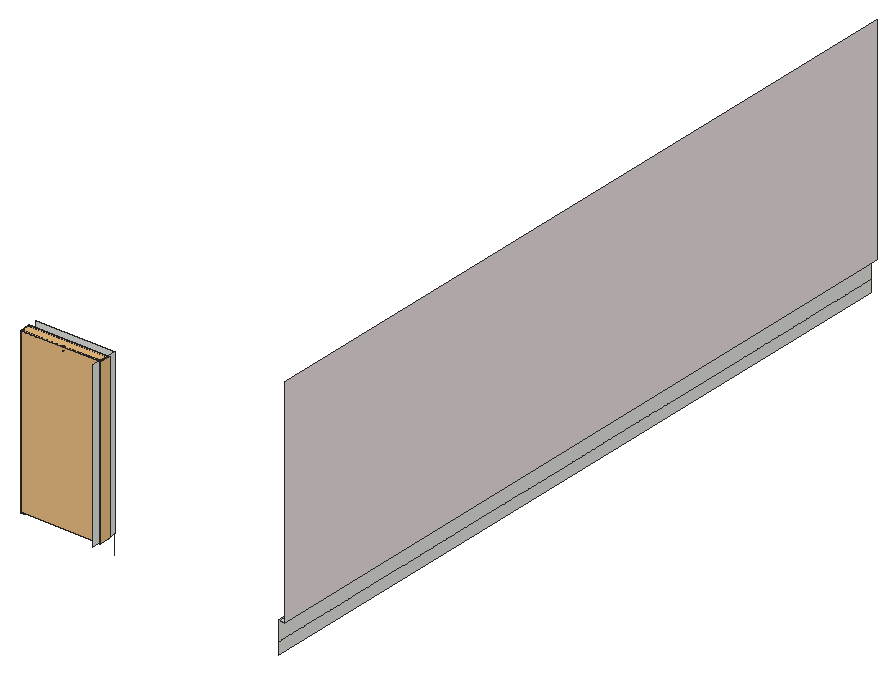
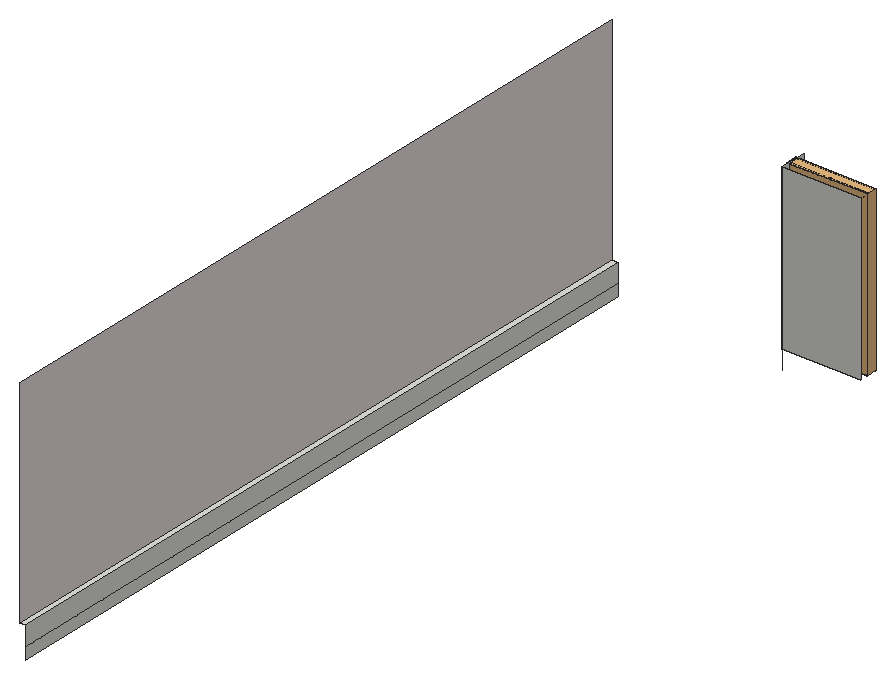
# SketchUp Ruby script. Lengths in inches.
U = 1.inch
M = Sketchup.active_model
def pt(a) = Geom::Point3d.new(a.map { |v| v * U })
def face(e, loops, mat)
  f = e.add_face(loops[0].map { |a| pt(a) })
  loops[1..].each { |l| e.add_face(l.map { |a| pt(a) }).erase! }
  f.material = f.back_material = mat if mat
  f
end
# faces: each face lists its corners as indices into pts; further lists are holes
def faces(e, pts, list, mat = nil) = list.each { |f| face(e, (f[0].is_a?(Array) ? f : [f]).map { |l| l.map { |i| pts[i] } }, mat) }
# xy, xz, yz: faces in a plane at the given z, y or x. An outline is a flat list of corners, or four numbers for a rectangle; further outlines are holes
def ring(l) = l.size == 4 ? [[l[0], l[1]], [l[2], l[1]], [l[2], l[3]], [l[0], l[3]]] : l.each_slice(2).to_a
def flat(e, list, mat, &to3) = list.each { |f| face(e, (f[0].is_a?(Array) ? f : [f]).map { |l| ring(l).map { |u, v| to3.(u, v) } }, mat) }
def xy(e, z, list, mat = nil) = flat(e, list, mat) { |x, y| [x, y, z] }
def xz(e, y, list, mat = nil) = flat(e, list, mat) { |x, z| [x, y, z] }
def yz(e, x, list, mat = nil) = flat(e, list, mat) { |y, z| [x, y, z] }
def lines(e, pts, list) = list.each { |a, b| e.add_line(pt(pts[a]), pt(pts[b])) }
# prism: a flat outline (further loops are holes) pulled along v
def prism(e, loops, v, mat = nil)
  f = face(e, loops, mat); d = Geom::Vector3d.new(v.map { |x| x * U })
  f.pushpull(f.normal.samedirection?(d) ? d.length : -d.length)
end
def box(e, o, s, mat = nil) = prism(e, [[o, [o[0] + s[0], o[1], o[2]], [o[0] + s[0], o[1] + s[1], o[2]], [o[0], o[1] + s[1], o[2]]]], [0, 0, s[2]], mat)
def at(x, y, z, deg = 0) = Geom::Transformation.translation(pt([x, y, z])) * Geom::Transformation.rotation(ORIGIN, Z_AXIS, deg.degrees)
def axes(o, x, y, z) = Geom::Transformation.new([*x, 0, *y, 0, *z, 0, *pt(o).to_a, 1])
def part(name) = M.definitions.add(name)
# library, detail: a bought-in or finely detailed component or shape, given as its bounding box
def library(name, o, s) = part(name).tap { |d| box(d.entities, o, s) }
def detail(e, o, s) = box(e.add_group.entities, o, s)
def put(e, d, t, mat = nil) = e.add_instance(d, t).tap { |i| i.material = mat if mat }
def group(e, t, mat = nil) = e.add_group.tap { |g| g.transformation = t; g.material = mat if mat }.entities
root = M.entities
M.materials.add("Generic\#9").color = [233, 223, 223]
M.materials.add("Material \#0").color = [86, 53, 35]
M.materials.add("Material \#1").color = [140, 140, 140]
c1 = part("3DGeom~19_Defintion")
xy(c1.entities,0,[[-6.28,-215.79,-994.45,-208.55,-13.52,-208.55],[-994.45,-215.79,-994.45,-208.55,-6.28,-215.79],[-6.28,-215.79,-13.52,-208.55,-13.52,0],[-6.28,-215.79,-13.52,0,-6.28,0],[-13.52,0,-13.52,208.55,-6.28,215.79],
  [-13.52,0,-6.28,215.79,-6.28,0],[-994.45,208.55,-6.28,215.79,-13.52,208.55],[-994.45,208.55,-994.45,215.79,-6.28,215.79]],"Material \#0")
p = [[-13.52,-208.55,0],[-994.45,-208.55,0],[-994.45,-207.81,0.07],[-14.25,-207.81,0.07],[-13.52,-208.55,0],[-14.25,-207.81,0.07],
  [-14.25,0,0.07],[-13.52,0,0],[-13.52,208.55,0],[-14.25,207.81,0.07],[-13.52,208.55,0],[-14.25,207.81,0.07],
  [-994.45,207.81,0.07],[-994.45,208.55,0],[-994.45,-207.21,0.27],[-994.45,-207.21,0.27],[-14.86,-207.21,0.27],[-14.86,-207.21,0.27],
  [-14.86,0,0.27],[-14.86,0,0.27],[-14.86,0,0.27],[-14.86,0,0.27],[-14.86,207.21,0.27],[-14.86,207.21,0.27],
  [-994.45,207.21,0.27],[-994.45,207.21,0.27],[-14.86,-207.21,0.27],[-994.45,-207.21,0.27],[-994.45,-206.74,0.6],[-15.33,-206.74,0.6],
  [-14.86,-207.21,0.27],[-15.33,-206.74,0.6],[-15.33,0,0.6],[-14.86,0,0.27],[-14.86,207.21,0.27],[-15.33,206.74,0.6],
  [-14.86,207.21,0.27],[-15.33,206.74,0.6],[-994.45,206.74,0.6],[-994.45,207.21,0.27],[-994.45,-206.4,1.07],[-15.66,-206.4,1.07],
  [-15.66,-206.4,1.07],[-15.66,0,1.07],[-15.66,206.4,1.07],[-15.66,206.4,1.07],[-994.45,206.4,1.07],[-994.45,-206.2,1.68],
  [-15.86,-206.2,1.68],[-15.86,-206.2,1.68],[-15.86,0,1.68],[-15.86,206.2,1.68],[-15.86,206.2,1.68],[-994.45,206.2,1.68],
  [-994.45,-206.13,2.41],[-15.93,-206.13,2.41],[-15.93,-206.13,2.41],[-15.93,0,2.41],[-15.93,206.13,2.41],[-15.93,206.13,2.41],
  [-994.45,206.13,2.41],[-994.45,-206.13,71.16],[-994.45,-206.22,71.59],[-15.79,-206.28,71.53],[-15.79,-206.28,71.53],[-15.84,0,71.59],
  [-15.93,0,71.16],[-15.79,206.28,71.53],[-15.79,206.28,71.53],[-994.45,206.22,71.59],[-994.45,206.13,71.16],[-15.79,-206.28,71.53],
  [-994.45,-206.48,71.84],[-994.45,-206.9,71.93],[-15.16,-206.9,71.93],[-15.79,-206.28,71.53],[-15.79,-206.28,71.53],[-15.16,-206.9,71.93],
  [-15.16,0,71.93],[-994.45,-206.48,71.84],[-15.59,0,71.84],[-15.79,-206.28,71.53],[-15.59,0,71.84],[-15.79,206.28,71.53],
  [-15.16,206.9,71.93],[-15.59,0,71.84],[-15.79,206.28,71.53],[-994.45,206.48,71.84],[-15.79,206.28,71.53],[-15.16,206.9,71.93],
  [-994.45,206.9,71.93],[-994.45,206.48,71.84],[-15.79,206.28,71.53],[-994.45,-227.27,72.01],[5.41,-227.47,72.33],[4.78,-226.84,71.93],
  [4.78,-226.84,71.93],[5.41,-227.47,72.33],[5.21,0,72.01],[-994.45,-226.84,71.93],[-994.45,-227.27,72.01],[5.21,0,72.01],
  [4.78,0,71.93],[4.78,226.84,71.93],[5.21,0,72.01],[5.21,0,72.01],[5.41,227.47,72.33],[4.78,226.84,71.93],
  [5.41,227.47,72.33],[-994.45,227.27,72.01],[-994.45,227.27,72.01],[-994.45,226.84,71.93],[-994.45,-227.27,72.01],[-994.45,-227.53,72.27],
  [5.41,-227.47,72.33],[5.41,-227.47,72.33],[5.47,0,72.27],[5.21,0,72.01],[5.41,227.47,72.33],[5.41,227.47,72.33],
  [-994.45,227.53,72.27],[-994.45,227.27,72.01],[-994.45,-227.61,72.7],[-994.45,-227.61,74.4375],[-994.45,-227.61,74.4375],[5.55,-227.61,74.4375],
  [5.55,-227.61,74.4375],[5.55,0,74.4375],[5.55,0,72.7],[5.55,227.61,74.4375],[5.55,227.61,74.4375],[-994.45,227.61,74.4375],
  [-994.45,227.61,74.4375],[-994.45,227.61,72.7]]
faces(c1.entities,p,[[0,1,2],[2,3,0],[4,5,6],[6,7,4],[8,7,6],[6,9,8],[10,11,12],[12,13,10],
  [3,2,14],[15,16,3],[5,17,18],[19,6,5],[9,6,20],[21,22,9],[11,23,24],[25,12,11],
  [26,27,28],[28,29,26],[30,31,32],[32,33,30],[34,33,32],[32,35,34],[36,37,38],[38,39,36],
  [29,28,40],[40,41,29],[31,42,43],[43,32,31],[35,32,43],[43,44,35],[37,45,46],[46,38,37],
  [41,40,47],[47,48,41],[42,49,50],[50,43,42],[44,43,50],[50,51,44],[45,52,53],[53,46,45],
  [48,47,54],[54,55,48],[49,56,57],[57,50,49],[51,50,57],[57,58,51],[52,59,60],[60,53,52],
  [61,62,63],[64,65,66],[66,65,67],[68,69,70],[71,72,73],[73,74,75],[76,77,78],[62,79,63],
  [78,80,76],[81,82,65],[83,80,78],[78,84,83],[65,85,86],[68,87,69],[88,89,90],[90,91,92],
  [93,94,95],[96,97,98],[95,99,100],[101,102,96],[103,102,104],[105,106,103],[107,108,109],[110,111,107],
  [112,113,114],[115,116,117],[117,116,118],[119,120,121],[114,122,123],[124,125,114],[113,122,114],[115,126,127],
  [127,128,115],[115,128,116],[118,128,127],[127,129,118],[116,128,118],[119,130,131],[132,133,119],[119,133,120]],"Material \#0")
c2 = part("3DGeom~15_Defintion")
xy(c2.entities,0,[[-961.58,-251.9,-958.5,-248.8125,-961.58,-237.8],[-961.58,-251.9,28.8,-248.8125,-958.5,-248.8125],[-961.58,-251.9,36.25,-251.9,28.8,-248.8125],[36.25,-251.9,19.98,-239.99,28.8,-248.8125],[36.25,-251.9,22.16,-237.8,19.98,-239.99],
  [-958.5,-248.8125,-958.5,-237.8,-961.58,-237.8],[19.98,-239.99,22.16,-237.8,3.36,-223.37],[-958.5,-237.8,-958.5,-223.37,-961.58,-220.28],[-961.58,-237.8,-958.5,-237.8,-961.58,-220.28],[22.16,-237.8,4.64,-220.28,3.36,-223.37],
  [-958.5,-223.37,4.64,-220.28,-961.58,-220.28],[-958.5,-223.37,3.36,-223.37,4.64,-220.28],[5.29,-219.63,8.375,-218.35,5.29,0],[8.375,-218.35,8.375,0,5.29,0],[5.29,0,8.375,0,5.29,219.63],
  [8.375,0,8.375,218.35,5.29,219.63],[8.375,218.35,22.8125,237.15,5.29,219.63],[-961.58,220.28,-958.5,223.37,-961.58,237.8],[-961.58,220.28,3.36,223.37,-958.5,223.37],[-961.58,220.28,4.64,220.28,3.36,223.37],
  [4.64,220.28,19.98,239.99,3.36,223.37],[4.64,220.28,22.16,237.8,19.98,239.99],[-958.5,223.37,-958.5,237.8,-961.58,237.8],[-958.5,237.8,-958.5,248.8125,-961.58,251.9],[-961.58,237.8,-958.5,237.8,-961.58,251.9],
  [22.16,237.8,28.8,248.8125,19.98,239.99],[22.16,237.8,36.25,251.9,28.8,248.8125],[-958.5,248.8125,36.25,251.9,-961.58,251.9],[-958.5,248.8125,28.8,248.8125,36.25,251.9]],"Material \#0")
xy(c2.entities,7.48,[[-962.79,-238.36,23.37,-238.36,-962.79,-219.67],[23.37,-238.36,4.67,-219.67,-962.79,-219.67],[23.37,-238.36,23.37,0,4.67,-219.67],[4.67,-219.67,23.37,0,4.67,0],[23.37,0,23.37,238.36,4.67,219.67],
  [4.67,0,23.37,0,4.67,219.67],[-962.79,219.67,23.37,238.36,-962.79,238.36],[-962.79,219.67,4.67,219.67,23.37,238.36]],"Material \#0")
xy(c2.entities,63.5625,[[-962.79,-238.36,-962.79,-219.67,4.67,-219.67],[-962.79,-238.36,4.67,-219.67,23.37,-238.36],[23.37,-238.36,4.67,-219.67,23.37,0],[4.67,-219.67,4.67,0,23.37,0],[23.37,0,4.67,219.67,23.37,238.36],
  [4.67,0,4.67,219.67,23.37,0],[-962.79,219.67,-962.79,238.36,4.67,219.67],[4.67,219.67,-962.79,238.36,23.37,238.36]],"Material \#0")
xy(c2.entities,69.64,[[-962.79,-219.62,4.63,-219.62,-962.79,-200.32],[4.63,-219.62,-14.68,-200.32,-962.79,-200.32],[4.63,-219.62,4.63,0,-14.68,-200.32],[-14.68,-200.32,4.63,0,-14.68,0],[-14.68,0,4.63,0,-14.68,200.32],
  [4.63,0,4.63,219.62,-14.68,200.32],[-962.79,200.32,-14.68,200.32,4.63,219.62],[-962.79,200.32,4.63,219.62,-962.79,219.62]],"Material \#0")
xy(c2.entities,71.04,[[-961.58,-251.9,-958.5,-248.8125,28.8,-248.8125],[-961.58,-251.9,-961.58,-237.8,-958.5,-248.8125],[-961.58,-251.9,28.8,-248.8125,36.25,-251.9],[36.25,-251.9,19.98,-239.99,22.16,-237.8],[36.25,-251.9,28.8,-248.8125,19.98,-239.99],
  [-958.5,-248.8125,-961.58,-237.8,-958.5,-237.8],[19.98,-239.99,3.36,-223.37,22.16,-237.8],[-958.5,-237.8,-961.58,-220.28,-958.5,-223.37],[-961.58,-237.8,-961.58,-220.28,-958.5,-237.8],[22.16,-237.8,3.36,-223.37,4.64,-220.28],
  [-958.5,-223.37,-961.58,-220.28,4.64,-220.28],[-958.5,-223.37,4.64,-220.28,3.36,-223.37],[5.29,-219.63,5.29,0,8.375,-218.35],[8.375,-218.35,5.29,0,8.375,0],[5.29,0,5.29,219.63,8.375,0],
  [8.375,0,5.29,219.63,8.375,218.35],[8.375,218.35,5.29,219.63,22.8125,237.15],[-961.58,220.28,-958.5,223.37,3.36,223.37],[-961.58,220.28,-961.58,237.8,-958.5,223.37],[-961.58,220.28,3.36,223.37,4.64,220.28],
  [4.64,220.28,3.36,223.37,19.98,239.99],[4.64,220.28,19.98,239.99,22.16,237.8],[-958.5,223.37,-961.58,237.8,-958.5,237.8],[-958.5,237.8,-961.58,251.9,-958.5,248.8125],[-961.58,237.8,-961.58,251.9,-958.5,237.8],
  [22.16,237.8,19.98,239.99,28.8,248.8125],[22.16,237.8,28.8,248.8125,36.25,251.9],[-958.5,248.8125,-961.58,251.9,36.25,251.9],[-958.5,248.8125,36.25,251.9,28.8,248.8125]],"Material \#0")
xz(c2.entities,-238.36,[[-962.79,63.5625,23.37,63.5625,23.37,72.07],[-962.79,63.5625,23.37,72.07,-962.79,72.07]],"Material \#0")
xz(c2.entities,-219.67,[[-962.79,7.48,4.67,7.48,-962.79,63.5625],[4.67,7.48,4.67,63.5625,-962.79,63.5625]],"Material \#0")
xz(c2.entities,219.67,[[-962.79,7.48,-962.79,63.5625,4.67,7.48],[4.67,7.48,-962.79,63.5625,4.67,63.5625]],"Material \#0")
xz(c2.entities,238.36,[[-962.79,63.5625,-962.79,72.07,23.37,72.07],[-962.79,63.5625,23.37,72.07,23.37,63.5625]],"Material \#0")
yz(c2.entities,4.67,[[-219.67,7.48,0,7.48,-219.67,63.5625],[0,7.48,0,63.5625,-219.67,63.5625],[0,7.48,219.67,63.5625,0,63.5625],[0,7.48,219.67,7.48,219.67,63.5625]],"Material \#0")
yz(c2.entities,23.37,[[-238.36,63.5625,0,63.5625,-238.36,72.07],[0,63.5625,0,72.07,-238.36,72.07],[0,63.5625,238.36,63.5625,238.36,72.07],[0,63.5625,238.36,72.07,0,72.07]],"Material \#0")
p = [[36.9,-251.24,0],[37.21,0,-0.16],[34.125,0,-0.14],[36.9,251.24,0],[33.83,243.81,0.02],[33.83,-243.8,0.02],
  [22.8125,-237.15,0],[24.99,-234.97,-0.01],[5.375,-220.37,0],[23.37,-238.36,7.48],[4.67,-219.67,7.48],[4.67,-219.67,7.48],
  [23.37,-238.36,7.48],[23.37,-238.36,0],[4.67,-219.67,7.48],[23.37,-238.36,0],[5.375,-220.37,0],[5.375,-220.37,0],
  [23.37,-238.36,0],[5.29,-219.63,0],[8.375,-218.35,0],[-15.36,-199.64,1.62],[4.67,-219.67,7.48],[5.375,-220.37,0],
  [-13.8,-201.19,0.06],[5.375,-220.37,0],[5.375,-220.37,0],[-14.84,-200.15,0.58],[5.375,-220.37,0],[-13.8,-201.19,0.06],
  [-6.08,-208.92,0],[5.375,-220.37,0],[-13.8,-201.19,0.06],[-6.08,-208.92,0],[-13.8,-201.19,0.06],[5.375,-220.37,0],
  [-6.08,-208.92,0],[-13.8,-201.19,0.06],[-13.09,-201.91,0],[-6.08,-208.92,0],[-13.09,-201.91,0],[-13.8,-201.19,0.06],
  [-15.36,199.64,1.62],[4.67,219.67,7.48],[5.375,220.37,0],[-13.8,201.19,0.06],[5.375,220.37,0],[5.375,220.37,0],
  [4.67,219.67,7.48],[-14.84,200.15,0.58],[5.375,220.37,0],[-13.8,201.19,0.06],[-6.08,208.92,0],[-13.09,201.91,0],
  [-13.8,201.19,0.06],[-6.08,208.92,0],[-13.8,201.19,0.06],[5.375,220.37,0],[-6.08,208.92,0],[5.375,220.37,0],
  [-13.8,201.19,0.06],[-6.08,208.92,0],[-13.8,201.19,0.06],[-13.09,201.91,0],[8.375,218.35,0],[24.99,234.97,-0.01],
  [22.8125,237.15,0],[23.37,238.36,7.48],[23.37,238.36,0],[23.37,238.36,0],[5.375,220.37,0],[5.375,220.37,0],
  [23.37,238.36,7.48],[4.67,219.67,7.48],[5.375,220.37,0],[23.37,238.36,0],[23.37,238.36,7.48],[-13.8,-201.19,0.06],
  [-14.84,-200.15,0.58],[-14.38,-200.61,0.26],[-13.8,-201.19,0.06],[-13.8,-201.19,0.06],[-14.38,-200.61,0.26],[-13.8,201.19,0.06],
  [-14.84,200.15,0.58],[-13.8,201.19,0.06],[-14.38,200.61,0.26],[-14.38,200.61,0.26],[-13.8,201.19,0.06],[4.63,-219.62,69.64],
  [4.63,-219.62,69.64],[-15.42,-199.57,9.43],[-15.36,-199.64,1.62],[-15.16,-199.83,1.04],[-15.16,-199.83,1.04],[-15.16,199.83,1.04],
  [-15.36,199.64,1.62],[-15.16,199.83,1.04],[-15.42,199.57,9.43],[4.63,219.62,69.64],[4.67,219.67,7.48],[4.63,219.62,69.64],
  [4.63,-219.62,69.64],[4.67,-219.67,63.5625],[4.67,-219.67,63.5625],[4.67,-219.67,7.48],[-15.28,-199.71,69.25],[4.63,-219.62,69.64],
  [-15.42,-199.57,9.43],[-15.28,-199.71,69.25],[-15.42,-199.57,2.34],[-15.42,-199.57,2.34],[-15.42,199.57,2.34],[-15.42,199.57,9.43],
  [-15.28,199.71,69.25],[-15.28,199.71,69.25],[4.63,219.62,69.64],[4.63,219.62,69.64],[4.67,219.67,63.5625],[4.67,219.67,63.5625],
  [-15.42,199.57,2.34],[4.67,-219.67,63.5625],[4.63,-219.62,69.64],[4.67,219.67,7.48],[4.67,219.67,63.5625],[4.63,219.62,69.64],
  [4.63,-219.62,69.64],[-15.28,-199.71,69.25],[-15.28,-199.71,69.25],[-15.42,-199.57,48.99],[-15.42,-199.57,48.99],[-15.28,-199.71,69.25],
  [-15.42,199.57,48.99],[-15.28,199.71,69.25],[-15.28,199.71,69.25],[-15.42,199.57,48.99],[4.63,219.62,69.64],[4.63,-219.62,69.64],
  [23.37,-238.36,72.07],[4.67,-219.67,63.5625],[4.67,-219.67,63.5625],[23.37,-238.36,63.5625],[23.37,-238.36,72.07],[4.67,-219.67,63.5625],
  [5.24,-220.23,70.03],[23.37,-238.36,72.07],[23.37,-238.36,63.5625],[4.67,-219.67,63.5625],[4.67,-219.67,63.5625],[4.63,-219.62,69.64],
  [4.63,219.62,69.64],[23.37,238.36,72.07],[4.67,219.67,63.5625],[4.67,219.67,63.5625],[5.24,220.23,70.03],[4.63,219.62,69.64],
  [23.37,238.36,63.5625],[4.67,219.67,63.5625],[4.67,219.67,63.5625],[23.37,238.36,63.5625],[23.37,238.36,72.07],[4.67,219.67,63.5625],
  [23.37,238.36,72.07],[4.63,-219.62,69.64],[-14.68,-200.32,69.64],[-15.28,-199.71,69.25],[-15.28,-199.71,69.25],[-14.68,-200.32,69.64],
  [4.63,-219.62,69.64],[-15.28,199.71,69.25],[-14.68,200.32,69.64],[4.63,219.62,69.64],[4.63,219.62,69.64],[-14.68,200.32,69.64],
  [4.63,-219.62,69.64],[5.24,-220.23,70.03],[23.37,-238.36,72.07],[4.63,219.62,69.64],[5.24,220.23,70.03],[5.375,-220.37,72.07],
  [5.375,-220.37,72.07],[23.37,-238.36,72.07],[5.375,220.37,72.07],[23.37,238.36,72.07],[5.375,220.37,72.07],[33.83,-243.8,71.03],
  [36.9,-251.24,71.04],[22.8125,-237.15,71.04],[34.125,0,71.19],[37.21,0,71.2],[24.99,-234.97,71.05],[5.29,-219.63,71.04],
  [8.375,-218.35,71.04],[33.83,243.81,71.03],[36.9,251.24,71.04],[22.8125,237.15,71.04],[24.99,234.97,71.05],[8.375,218.35,71.04]]
faces(c2.entities,p,[[0,1,2],[1,3,4],[4,2,1],[2,5,0],[6,0,5],[5,7,6],[8,9,10],[11,12,13],
  [14,15,16],[17,18,9],[19,6,7],[7,20,19],[21,22,23],[24,21,25],[26,10,27],[28,27,29],
  [30,31,32],[33,34,35],[36,37,38],[39,40,41],[42,43,44],[45,42,46],[47,48,49],[50,49,51],
  [52,53,54],[55,56,57],[58,59,60],[61,62,63],[64,65,66],[43,67,68],[43,69,70],[71,72,73],
  [74,75,76],[3,66,65],[65,4,3],[77,78,21],[27,79,80],[81,82,78],[83,84,42],[85,86,84],
  [49,87,88],[10,89,27],[90,91,27],[92,93,27],[91,92,27],[78,94,21],[84,95,42],[96,97,49],
  [98,96,49],[99,98,49],[100,101,49],[21,102,103],[21,104,105],[21,106,107],[21,108,109],[91,110,92],
  [21,111,108],[42,112,113],[42,113,114],[42,115,116],[42,117,118],[42,119,43],[98,120,96],[10,121,122],
  [123,124,125],[126,127,91],[128,129,91],[108,130,131],[113,132,133],[134,135,98],[136,134,98],[137,138,139],
  [140,141,142],[143,142,144],[145,146,147],[148,144,149],[150,151,152],[153,154,155],[151,156,157],[158,159,160],
  [161,162,154],[163,164,165],[166,167,168],[169,170,171],[172,173,134],[174,175,176],[177,178,151],[142,179,144],
  [175,180,181],[178,182,151],[183,184,154],[185,186,187],[186,185,188],[188,189,186],[187,190,185],[190,187,191],
  [191,192,190],[189,188,193],[193,194,189],[195,196,197],[196,195,194],[194,193,196]],"Material \#0")
c3 = part("3DGeom~22_Defintion")
xz(c3.entities,-210.625,[[-1016.13,2.47,-1016.13,9.96,-16.28,2.47],[-16.28,2.47,-1016.13,9.96,-16.28,9.96],[-1016.13,9.96,-1016.13,51.7,-16.28,51.7],[-1016.13,9.96,-16.28,51.7,-16.28,9.96],[-1016.13,51.7,-1016.13,72.71,-16.28,51.7]],"Material \#0")
xz(c3.entities,210.625,[[-1016.13,2.47,-16.28,2.47,-1016.13,9.96],[-16.28,2.47,-16.28,9.96,-1016.13,9.96],[-1016.13,9.96,-16.28,51.7,-1016.13,51.7],[-1016.13,9.96,-16.28,9.96,-16.28,51.7],[-1016.13,51.7,-16.28,51.7,-1016.13,72.71]],"Material \#0")
yz(c3.entities,-16.28,[[-210.625,2.47,-210.625,9.96,0,9.96],[-210.625,2.47,0,9.96,0,2.47],[0,2.47,0,9.96,210.625,2.47],[210.625,2.47,0,9.96,210.625,9.96],[-210.625,9.96,-210.625,51.7,0,51.7],
  [-210.625,9.96,0,51.7,0,9.96],[0,9.96,0,51.7,210.625,9.96],[210.625,9.96,0,51.7,210.625,51.7],[-210.625,51.7,0,72.71,0,51.7],[0,51.7,0,72.71,210.625,51.7]],"Material \#0")
p = [[-1016.13,-210.625,72.71],[-16.13,-210.77,73.09],[-16.28,-210.625,51.7],[-16.28,-210.625,51.7],[-16.13,-210.77,73.09],[-16.28,0,72.71],
  [-16.13,210.77,73.09],[-16.28,210.625,51.7],[-16.28,210.625,51.7],[-16.13,210.77,73.09],[-1016.13,210.625,72.71]]
faces(c3.entities,p,[[0,1,2],[3,4,5],[5,6,7],[8,9,10]],"Material \#0")
c4 = library("3DGeom~16_Defintion",[-962.62,-252.34,-11.22],[1000,504.68,93.46])
c5 = part("3DGeom~17_Defintion")
yz(c5.entities,-1908.8,[[-436.03,-21.87,-436.73,-21.5,-435.91,-21.83],[436.03,-21.87,435.91,-21.83,436.73,-21.5],[-435.91,-21.83,-436.73,-21.5,-436.15,-21.125],[-435.91,-21.83,-436.15,-21.125,-435.87,-21.72],[435.91,-21.83,435.87,-21.72,436.15,-21.125],
  [435.91,-21.83,436.15,-21.125,436.73,-21.5],[-436.73,-21.5,-484.73,-21.37,-436.15,-1.11],[-471.46,-21.5,-484.73,-21.37,-436.73,-21.5],[-477.2,-21.5,-484.73,-21.37,-471.46,-21.5],[-481.82,-21.5,-484.73,-21.37,-477.2,-21.5],
  [-436.73,-21.5,-436.15,-1.11,-436.15,-21.125],[436.73,-21.5,436.15,-21.125,471.46,-21.5],[471.46,-21.5,436.15,-21.125,477.2,-21.5],[477.2,-21.5,436.15,-21.125,499.98,-0.85],[477.2,-21.5,499.98,-0.85,481.82,-21.5],
  [481.82,-21.5,487.35,-21,484.73,-21.37],[481.82,-21.5,491.8,-19.52,487.35,-21],[481.82,-21.5,497.64,-13.67,491.8,-19.52],[481.82,-21.5,499.98,-0.85,497.64,-13.67],[-484.73,-21.37,-498.5,-11.58,-499.84,-0.37],
  [-484.73,-21.37,-499.84,-0.37,-499.4,-0.5],[-484.73,-21.37,-499.4,-0.5,-436.15,-1.11],[-484.73,-21.37,-493.63,-18.42,-498.5,-11.58],[-484.73,-21.37,-489.71,-20.375,-493.63,-18.42],[-484.73,-21.37,-487.35,-21,-489.71,-20.375],
  [436.15,-21.125,436.15,-1.11,436.73,-0.74],[436.15,-21.125,436.73,-0.74,499.98,-0.85],[487.35,-21,491.8,-19.52,489.71,-20.375],[-489.71,-20.375,-491.8,-19.52,-493.63,-18.42],[491.8,-19.52,495.21,-17.08,493.63,-18.42],
  [491.8,-19.52,497.64,-13.67,495.21,-17.08],[-493.63,-18.42,-496.54,-15.5,-498.5,-11.58],[-493.63,-18.42,-495.21,-17.08,-496.54,-15.5],[495.21,-17.08,497.64,-13.67,496.54,-15.5],[-496.54,-15.5,-497.64,-13.67,-498.5,-11.58],
  [497.64,-13.67,499.125,-9.22,498.5,-11.58],[497.64,-13.67,499.625,-3.69,499.125,-9.22],[497.64,-13.67,499.98,-0.85,499.625,-3.69],[-498.5,-11.58,-499.625,-3.69,-499.84,-0.37],[-498.5,-11.58,-499.5,-6.6,-499.625,-3.69],
  [-498.5,-11.58,-499.125,-9.22,-499.5,-6.6],[499.125,-9.22,499.625,-3.69,499.5,-6.6],[-499.625,-3.69,-499.98,-0.85,-500,-0.52],[-499.625,-3.69,-500,-0.52,-499.84,-0.37],[-436.15,-1.11,-499.4,-0.5,-471.46,-0.74],
  [-436.15,-1.11,-471.46,-0.74,-436.73,-0.74],[-436.15,-1.11,-436.73,-0.74,-435.91,-0.41],[-436.15,-1.11,-435.91,-0.41,-435.87,-0.52],[436.15,-1.11,435.87,-0.52,435.91,-0.41],[436.15,-1.11,435.91,-0.41,436.73,-0.74],
  [499.98,-0.85,436.73,-0.74,471.46,-0.74],[499.98,-0.85,471.46,-0.74,499.4,-0.5],[499.98,-0.85,499.4,-0.5,499.96,-0.41],[499.98,-0.85,499.96,-0.41,500,-0.52],[-436.73,-0.74,-436.03,-0.37,-435.91,-0.41],
  [436.73,-0.74,435.91,-0.41,436.03,-0.37],[-500,-0.52,-499.96,-0.41,-499.84,-0.37],[499.4,-0.5,499.84,-0.37,499.96,-0.41],[-499.84,141.21,-499.96,141.25,-499.4,141.35],[-436.03,141.21,-436.73,141.59,-435.91,141.25],
  [436.03,141.21,435.91,141.25,436.73,141.59],[499.84,141.21,484.73,162.21,498.5,152.42],[499.84,141.21,499.4,141.35,484.73,162.21],[499.84,141.21,498.5,152.42,499.625,144.53],[499.84,141.21,499.625,144.53,500,141.37],
  [499.84,141.21,500,141.37,499.96,141.25],[-499.96,141.25,-500,141.37,-499.98,141.69],[-499.96,141.25,-499.98,141.69,-499.4,141.35],[-435.91,141.25,-436.73,141.59,-436.15,141.96],[-435.91,141.25,-436.15,141.96,-435.87,141.37],
  [435.91,141.25,435.87,141.37,436.15,141.96],[435.91,141.25,436.15,141.96,436.73,141.59],[-499.4,141.35,-499.98,141.69,-471.46,141.59],[499.4,141.35,436.15,141.96,484.73,162.21],[499.4,141.35,471.46,141.59,436.15,141.96],
  [500,141.37,499.625,144.53,499.98,141.69],[-436.73,141.59,-499.98,141.69,-436.15,161.97],[-471.46,141.59,-499.98,141.69,-436.73,141.59],[-436.73,141.59,-436.15,161.97,-436.15,141.96],[436.73,141.59,436.15,141.96,471.46,141.59],
  [-499.98,141.69,-477.2,162.34,-436.15,161.97],[-499.98,141.69,-481.82,162.34,-477.2,162.34],[-499.98,141.69,-497.64,154.51,-481.82,162.34],[-499.98,141.69,-499.625,144.53,-497.64,154.51],[436.15,141.96,436.15,161.97,436.73,162.34],
  [436.15,141.96,436.73,162.34,484.73,162.21],[-499.625,144.53,-499.125,150.07,-497.64,154.51],[-499.625,144.53,-499.5,147.44,-499.125,150.07],[499.625,144.53,498.5,152.42,499.5,147.44],[499.5,147.44,498.5,152.42,499.125,150.07],
  [-499.125,150.07,-498.5,152.42,-497.64,154.51],[498.5,152.42,484.73,162.21,493.63,159.26],[498.5,152.42,493.63,159.26,496.54,156.34],[498.5,152.42,496.54,156.34,497.64,154.51],[-497.64,154.51,-491.8,160.36,-481.82,162.34],
  [-497.64,154.51,-495.21,157.92,-491.8,160.36],[-497.64,154.51,-496.54,156.34,-495.21,157.92],[496.54,156.34,493.63,159.26,495.21,157.92],[-495.21,157.92,-493.63,159.26,-491.8,160.36],[493.63,159.26,484.73,162.21,489.71,161.22],
  [493.63,159.26,489.71,161.22,491.8,160.36],[-491.8,160.36,-487.35,161.84,-481.82,162.34],[-491.8,160.36,-489.71,161.22,-487.35,161.84],[489.71,161.22,484.73,162.21,487.35,161.84],[-487.35,161.84,-484.73,162.21,-481.82,162.34],
  [-436.15,161.97,-477.2,162.34,-471.46,162.34],[-436.15,161.97,-471.46,162.34,-436.73,162.34],[-436.15,161.97,-436.73,162.34,-435.91,162.68],[-436.15,161.97,-435.91,162.68,-435.87,162.56],[436.15,161.97,435.87,162.56,435.91,162.68],
  [436.15,161.97,435.91,162.68,436.73,162.34],[484.73,162.21,436.73,162.34,471.46,162.34],[484.73,162.21,471.46,162.34,477.2,162.34],[484.73,162.21,477.2,162.34,481.82,162.34],[-436.73,162.34,-436.03,162.72,-435.91,162.68],
  [436.73,162.34,435.91,162.68,436.03,162.72]],"Material \#0")
c6 = part("3DGeom~18_Defintion")
xz(c6.entities,-241.71,[[-976.3,0,23.7,0,23.7,7.58],[-976.3,0,23.7,7.58,-976.3,7.58]],"Material \#0")
xz(c6.entities,241.71,[[-976.3,0,-976.3,7.58,23.7,7.58],[-976.3,0,23.7,7.58,23.7,0]],"Material \#0")
yz(c6.entities,23.7,[[-241.71,0,0,0,-241.71,7.58],[0,0,0,7.58,-241.71,7.58],[0,0,241.71,0,241.71,7.58],[0,0,241.71,7.58,0,7.58]],"Material \#0")
c7 = part("3DGeom~20_Defintion")
xy(c7.entities,0,[[-976.3,-241.71,-976.3,-223.46,23.7,-241.71],[23.7,-241.71,-976.3,-223.46,5.45,-223.46],[23.7,-241.71,5.45,-223.46,5.45,0],[23.7,-241.71,5.45,0,23.7,0],[-976.3,-223.46,-976.3,-211.85,5.45,-223.46],
  [5.45,-223.46,-976.3,-211.85,-6.16,-211.85],[5.45,-223.46,-6.16,-211.85,-6.16,0],[5.45,-223.46,-6.16,0,5.45,0],[-6.16,0,-6.16,211.85,5.45,223.46],[-6.16,0,5.45,223.46,5.45,0],
  [5.45,0,23.7,241.71,23.7,0],[5.45,0,5.45,223.46,23.7,241.71],[-976.3,211.85,-976.3,223.46,5.45,223.46],[-976.3,211.85,5.45,223.46,-6.16,211.85],[-976.3,223.46,-976.3,241.71,23.7,241.71],
  [-976.3,223.46,23.7,241.71,5.45,223.46]],"Material \#0")
xy(root,0,[[488.6875,194.8125,491.875,607.4375]])
xz(root,201.113,[[347.824,37.502,347.952,37.526,347.824,37.514],[347.824,37.502,347.954,37.514,347.952,37.526],[347.954,37.514,348.072,37.56,347.952,37.526],[347.954,37.514,348.076,37.548,348.072,37.56],[348.076,37.548,348.183,37.614,348.072,37.56],
  [348.076,37.548,348.189,37.603,348.183,37.614],[348.189,37.603,348.282,37.686,348.183,37.614],[348.189,37.603,348.291,37.676,348.282,37.686],[348.291,37.676,348.368,37.774,348.282,37.686],[348.291,37.676,348.378,37.766,348.368,37.774],
  [347.824,37.7,347.865,37.717,347.824,37.713],[347.824,37.7,347.867,37.704,347.865,37.717],[347.867,37.704,347.903,37.728,347.865,37.717],[347.867,37.704,347.908,37.716,347.903,37.728],[347.908,37.716,347.939,37.745,347.903,37.728],
  [347.908,37.716,347.945,37.734,347.939,37.745],[347.945,37.734,347.971,37.768,347.939,37.745],[347.945,37.734,347.979,37.759,347.971,37.768],[347.979,37.759,347.998,37.796,347.971,37.768],[347.979,37.759,348.008,37.788,347.998,37.796],
  [348.008,37.788,348.021,37.829,347.998,37.796],[348.008,37.788,348.032,37.823,348.021,37.829],[348.032,37.823,348.038,37.866,348.021,37.829],[348.061,37.903,348.052,37.947,348.048,37.905],[348.061,37.903,348.065,37.947,348.052,37.947],
  [348.052,37.947,348.065,37.947,348.048,37.989],[348.038,38.029,348.049,38.033,348.021,38.065],[348.049,38.033,348.032,38.072,348.021,38.065],[348.021,38.065,348.032,38.072,347.998,38.098],[348.032,38.072,348.008,38.106,347.998,38.098],
  [347.998,38.098,348.008,38.106,347.971,38.126],[348.008,38.106,347.979,38.136,347.971,38.126],[347.971,38.126,347.979,38.136,347.939,38.149],[347.979,38.136,347.945,38.16,347.939,38.149],[347.939,38.149,347.945,38.16,347.903,38.167],
  [347.945,38.16,347.908,38.179,347.903,38.167],[347.903,38.167,347.908,38.179,347.865,38.178],[347.865,38.178,347.867,38.19,347.824,38.181],[347.865,38.178,347.908,38.179,347.867,38.19],[347.824,38.181,347.867,38.19,347.824,38.194]],"Material \#1")
xz(root,201.144,[[347.824,40.059,347.86,40.064,347.893,40.076],[347.824,40.059,347.893,40.076,347.947,40.12],[347.893,40.076,347.922,40.095,347.947,40.12],[347.947,40.12,347.824,40.539,347.767,40.546],[347.947,40.12,347.981,40.221,347.824,40.539],
  [347.947,40.12,347.965,40.15,347.977,40.184],[347.947,40.12,347.977,40.184,347.981,40.221],[347.981,40.221,347.881,40.546,347.824,40.539],[347.981,40.221,347.933,40.565,347.881,40.546],[347.981,40.221,347.979,40.595,347.933,40.565],
  [347.981,40.221,347.981,40.53,347.979,40.595],[347.981,40.53,347.983,40.543,347.979,40.595],[347.981,40.53,347.982,40.537,347.983,40.543],[347.983,40.543,348.018,40.635,347.979,40.595],[347.983,40.543,347.985,40.549,347.988,40.555],
  [347.983,40.543,347.988,40.555,348.018,40.635],[347.988,40.555,347.991,40.56,348.103,40.756],[347.988,40.555,348.047,40.682,348.018,40.635],[347.988,40.555,348.103,40.756,348.047,40.682],[347.991,40.56,347.995,40.565,348.103,40.756],
  [347.995,40.565,348,40.57,348.048,40.623],[347.995,40.565,348.048,40.623,348.103,40.756],[348,40.57,348.026,40.595,348.048,40.623],[348.048,40.623,348.068,40.653,348.084,40.685],[348.048,40.623,348.084,40.685,348.103,40.756],
  [348.047,40.682,348.103,40.756,348.066,40.736],[348.084,40.685,348.096,40.72,348.103,40.756],[348.066,40.736,348.103,40.756,348.072,40.794],[348.103,40.756,348.044,40.975,348.047,40.906],[348.103,40.756,348.098,40.861,348.044,40.975],
  [348.103,40.756,348.047,40.906,348.066,40.853],[348.103,40.756,348.066,40.853,348.072,40.794],[348.103,40.756,348.105,40.794,348.098,40.861],[348.098,40.861,348.077,40.921,348.044,40.975],[348.047,40.906,348.044,40.975,348.018,40.954],
  [348.018,40.954,348.044,40.975,347.979,40.993],[348.044,40.975,347.824,41.083,347.933,41.023],[348.044,40.975,347.948,41.054,347.824,41.083],[348.044,40.975,347.933,41.023,347.979,40.993],[348.044,40.975,348,41.02,347.948,41.054],
  [347.933,41.023,347.824,41.083,347.881,41.043],[347.881,41.043,347.824,41.083,347.824,41.049],[347.948,41.054,347.888,41.076,347.824,41.083]],"Material \#1")
xz(root,210.0625,[[340.778,0,384.716,90.9375]])
yz(root,384.716,[[194.8125,0,210.0625,90.9375]])
yz(root,488.6875,[[194.8125,-17.3125,607.4375,-10.875],[194.8125,-10.875,607.4375,0]])
yz(root,491.875,[[194.8125,0,607.4375,120]],"Generic\#9")
p = [[384.716,210.0625,0],[384.716,210.0625,-10.875]]
lines(root,p,[[0,1]])
put(root,c1,axes([363.16,204.75,87.54],[0,0,0.08803],[0.08585,0,0],[0,-0.06445,0]),"Material \#0")
put(root,c2,axes([363.16,204.75,87.54],[0,0,0.09092],[0.08867,0,0],[0,-0.06657,0]),"Material \#0")
put(root,c3,axes([363.16,204.75,87.54],[0,0,0.08615],[0.08402,0,0],[0,-0.06308,0]),"Material \#0")
put(root,c4,axes([363.16,204.75,87.54],[0,0,0.09094],[0.08869,0,0],[0,-0.06658,0]),"Material \#0")
put(root,c5,axes([363.16,204.75,87.54],[0,0,0.04586],[0.04473,0,0],[0,-0.03358,0]),"Material \#0")
put(root,c6,axes([363.16,204.75,87.54],[0,0,0.08966],[0.08745,0,0],[0,-0.06565,0]),"Material \#0")
put(root,c7,axes([363.16,204.75,87.54],[0,0,0.08966],[0.08745,0,0],[0,-0.06565,0]),"Material \#0")
